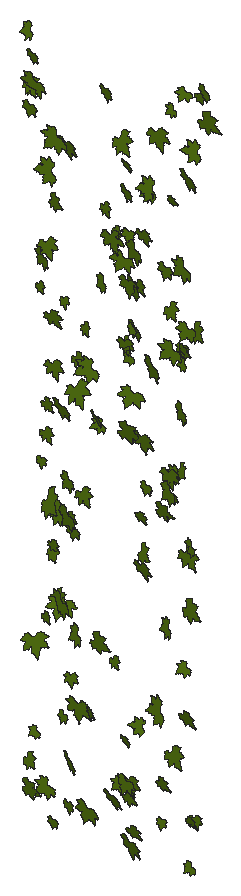
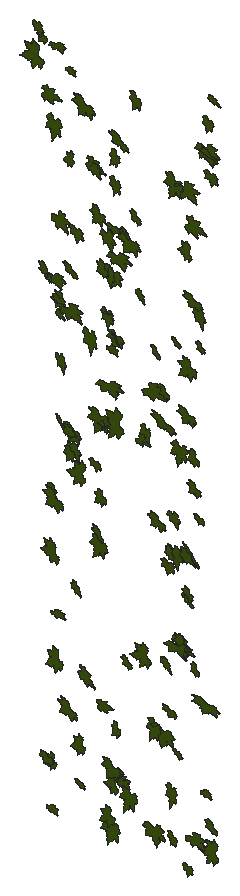
# SketchUp Ruby script. Lengths in inches.
U = 1.inch
M = Sketchup.active_model
def pt(a) = Geom::Point3d.new(a.map { |v| v * U })
def face(e, loops, mat)
  f = e.add_face(loops[0].map { |a| pt(a) })
  loops[1..].each { |l| e.add_face(l.map { |a| pt(a) }).erase! }
  f.material = f.back_material = mat if mat
  f
end
# faces: each face lists its corners as indices into pts; further lists are holes
def faces(e, pts, list, mat = nil) = list.each { |f| face(e, (f[0].is_a?(Array) ? f : [f]).map { |l| l.map { |i| pts[i] } }, mat) }
# xy, xz, yz: faces in a plane at the given z, y or x. An outline is a flat list of corners, or four numbers for a rectangle; further outlines are holes
def ring(l) = l.size == 4 ? [[l[0], l[1]], [l[2], l[1]], [l[2], l[3]], [l[0], l[3]]] : l.each_slice(2).to_a
def flat(e, list, mat, &to3) = list.each { |f| face(e, (f[0].is_a?(Array) ? f : [f]).map { |l| ring(l).map { |u, v| to3.(u, v) } }, mat) }
def xy(e, z, list, mat = nil) = flat(e, list, mat) { |x, y| [x, y, z] }
def xz(e, y, list, mat = nil) = flat(e, list, mat) { |x, z| [x, y, z] }
def yz(e, x, list, mat = nil) = flat(e, list, mat) { |y, z| [x, y, z] }
def lines(e, pts, list) = list.each { |a, b| e.add_line(pt(pts[a]), pt(pts[b])) }
# prism: a flat outline (further loops are holes) pulled along v
def prism(e, loops, v, mat = nil)
  f = face(e, loops, mat); d = Geom::Vector3d.new(v.map { |x| x * U })
  f.pushpull(f.normal.samedirection?(d) ? d.length : -d.length)
end
def box(e, o, s, mat = nil) = prism(e, [[o, [o[0] + s[0], o[1], o[2]], [o[0] + s[0], o[1] + s[1], o[2]], [o[0], o[1] + s[1], o[2]]]], [0, 0, s[2]], mat)
def at(x, y, z, deg = 0) = Geom::Transformation.translation(pt([x, y, z])) * Geom::Transformation.rotation(ORIGIN, Z_AXIS, deg.degrees)
def axes(o, x, y, z) = Geom::Transformation.new([*x, 0, *y, 0, *z, 0, *pt(o).to_a, 1])
def part(name) = M.definitions.add(name)
# library, detail: a bought-in or finely detailed component or shape, given as its bounding box
def library(name, o, s) = part(name).tap { |d| box(d.entities, o, s) }
def detail(e, o, s) = box(e.add_group.entities, o, s)
def put(e, d, t, mat = nil) = e.add_instance(d, t).tap { |i| i.material = mat if mat }
def group(e, t, mat = nil) = e.add_group.tap { |g| g.transformation = t; g.material = mat if mat }.entities
root = M.entities
M.materials.add("[Vegetation Blur 03]").color = [83, 114, 18]
c1 = part("ivy")
xy(c1.entities,0,[[0.782,0,0.786,0,0.787,0.005,0.789,0.009,0.821,0.072,0.875,0.147,1.001,0.272,1.073,0.331,1.137,0.363,1.178,0.379,1.223,0.384,1.272,0.383,1.311,0.374,1.36,0.355,1.399,0.334,1.491,0.285,1.541,0.244,1.583,0.199,1.617,0.15,1.64,0.128,1.662,0.115,1.717,0.105,1.745,0.093,1.784,0.054,1.819,0.057,1.854,0.064,1.882,0.075,1.896,0.074,1.91,0.071,1.937,0.063,1.964,0.053,1.99,0.038,2.016,0.015,2.034,0.002,2.04,0,2.038,0.003,2.036,0.007,2.033,0.038,2.036,0.068,2.045,0.1,2.055,0.116,2.064,0.123,2.077,0.129,2.088,0.129,2.106,0.132,2.118,0.13,2.179,0.132,2.207,0.133,2.225,0.133,2.242,0.138,2.22,0.162,2.207,0.186,2.206,0.213,2.212,0.236,2.228,0.262,2.247,0.274,2.298,0.283,2.355,0.294,2.37,0.296,2.376,0.295,2.377,0.3,2.377,0.303,2.385,0.329,2.411,0.37,2.426,0.392,2.449,0.407,2.511,0.426,2.561,0.444,2.619,0.466,2.589,0.469,2.561,0.476,2.501,0.5,2.449,0.516,2.424,0.523,2.401,0.535,2.377,0.556,2.372,0.568,2.36,0.575,2.268,0.586,2.225,0.592,2.207,0.599,2.194,0.61,2.143,0.65,2.13,0.664,2.122,0.682,2.123,0.7,2.13,0.719,2.148,0.75,2.17,0.781,2.195,0.807,2.221,0.828,2.284,0.874,2.291,0.88,2.288,0.887,2.276,0.9,2.267,0.916,2.265,0.933,2.273,0.967,2.292,1.002,2.313,1.03,2.334,1.054,2.348,1.067,2.358,1.074,2.363,1.076,2.362,1.081,2.35,1.094,2.347,1.11,2.35,1.143,2.359,1.18,2.385,1.254,2.415,1.324,2.448,1.393,2.45,1.4,2.446,1.398,2.44,1.394,2.427,1.383,2.402,1.36,2.376,1.339,2.345,1.324,2.305,1.309,2.282,1.303,2.273,1.306,2.245,1.294,2.212,1.287,2.187,1.291,2.163,1.301,2.142,1.316,2.134,1.327,2.124,1.325,2.09,1.292,2.053,1.259,2.014,1.234,1.973,1.215,1.954,1.21,1.931,1.208,1.909,1.212,1.893,1.22,1.879,1.233,1.872,1.248,1.867,1.281,1.864,1.319,1.821,1.258,1.773,1.197,1.726,1.141,1.698,1.121,1.679,1.116,1.666,1.117,1.647,1.122,1.632,1.129,1.62,1.141,1.617,1.154,1.617,1.219,1.621,1.254,1.623,1.268,1.623,1.281,1.618,1.314,1.606,1.346,1.603,1.375,1.607,1.403,1.603,1.467,1.599,1.499,1.605,1.525,1.614,1.552,1.629,1.577,1.635,1.589,1.629,1.587,1.618,1.582,1.596,1.566,1.581,1.556,1.568,1.552,1.557,1.55,1.545,1.553,1.531,1.562,1.522,1.572,1.504,1.591,1.486,1.611,1.474,1.631,1.457,1.666,1.455,1.684,1.457,1.698,1.452,1.715,1.444,1.728,1.424,1.754,1.419,1.772,1.423,1.786,1.434,1.819,1.444,1.848,1.446,1.855,1.44,1.861,1.43,1.867,1.386,1.904,1.349,1.948,1.326,1.973,1.31,1.995,1.288,2.048,1.284,2.153,1.287,2.254,1.284,2.255,1.282,2.253,1.278,2.247,1.274,2.237,1.266,2.216,1.226,2.125,1.208,2.076,1.184,2.033,1.155,1.984,1.135,1.942,1.111,1.899,1.083,1.861,1.053,1.85,1.059,1.83,1.061,1.809,1.056,1.79,1.049,1.767,1.04,1.749,1.018,1.733,0.994,1.726,0.942,1.734,0.95,1.6875,0.944,1.645,0.932,1.608,0.911,1.585,0.881,1.58,0.854,1.582,0.828,1.588,0.785,1.618,0.773,1.625,0.775,1.614,0.779,1.598,0.796,1.502,0.818,1.402,0.861,1.283,0.882,1.224,0.894,1.174,0.892,1.148,0.886,1.123,0.881,1.107,0.872,1.099,0.849,1.094,0.818,1.092,0.789,1.098,0.762,1.107,0.753,1.113,0.721,1.139,0.698,1.163,0.678,1.194,0.665,1.224,0.628,1.28,0.612,1.312,0.606,1.327,0.606,1.314,0.599,1.282,0.594,1.267,0.581,1.256,0.544,1.245,0.512,1.244,0.473,1.249,0.444,1.256,0.382,1.288,0.339,1.306,0.324,1.316,0.317,1.324,0.309,1.326,0.27,1.314,0.227,1.313,0.185,1.3125,0.152,1.317,0.122,1.328,0.092,1.345,0.073,1.353,0.079,1.338,0.092,1.308,0.117,1.249,0.13,1.215,0.139,1.164,0.147,1.148,0.157,1.136,0.163,1.122,0.174,1.086,0.177,1.067,0.182,1.054,0.186,1.043,0.191,1.038,0.211,1.028,0.237,1.005,0.25,0.974,0.253,0.96,0.25,0.944,0.242,0.914,0.243,0.906,0.249,0.902,0.26,0.894,0.289,0.88,0.307,0.873,0.322,0.862,0.364,0.799,0.403,0.738,0.431,0.709,0.439,0.691,0.441,0.678,0.4375,0.66,0.428,0.645,0.394,0.623,0.303,0.594,0.255,0.581,0.214,0.577,0.179,0.573,0.173,0.568,0.175,0.561,0.167,0.55,0.141,0.523,0.113,0.503,0.077,0.49,0.045,0.486,0.026,0.485,0.019,0.486,0.011,0.483,0,0.471,0.014,0.467,0.044,0.455,0.058,0.447,0.07,0.438,0.097,0.411,0.125,0.394,0.158,0.377,0.174,0.366,0.182,0.359,0.185,0.361,0.242,0.331,0.253,0.316,0.258,0.303,0.262,0.283,0.274,0.278,0.308,0.274,0.341,0.252,0.366,0.226,0.366,0.222,0.37,0.22,0.38,0.221,0.395,0.221,0.425,0.216,0.45,0.207,0.465,0.192,0.473,0.178,0.484,0.15,0.489,0.116,0.483,0.089,0.468,0.058,0.45,0.035,0.435,0.018,0.429,0.011,0.434,0.012,0.438,0.014,0.469,0.019,0.542,0.016,0.581,0.015,0.612,0.027,0.68,0.055,0.696,0.057,0.712,0.052,0.73,0.045,0.741,0.036,0.766,0.014]])
put(root,c1,axes([22.26,173.7,49.1875],[0.2034,-0.19719,-0.25526],[-0.32297,-0.00076,-0.17132],[-0.05192,-0.76775,0.06573]),"[Vegetation Blur 03]")
put(root,c1,axes([21.79,173.7,44.77],[0.4277,-0.13208,-0.01923],[-0.02433,-0.00684,-0.35292],[-0.0639,-0.88143,0.00562]),"[Vegetation Blur 03]")
put(root,c1,axes([21.72,173.7,8.45],[0.18478,0.02807,0.2907],[0.35178,-0.14758,-0.1467],[-0.05752,-0.81244,0.03669]),"[Vegetation Blur 03]")
put(root,c1,axes([21.94,173.7,46.46],[0.60025,-0.11632,-0.20653],[-0.25299,0.02521,-0.49198],[-0.05685,-1.34025,0.00867]),"[Vegetation Blur 03]")
put(root,c1,axes([21.68,173.7,45.55],[0.34233,0.0367,0.25351],[0.30852,-0.16299,-0.27378],[-0.04025,-0.93715,0.05755]),"[Vegetation Blur 03]")
put(root,c1,axes([21.74,173.7,6.73],[0.10484,-0.11239,0.45286],[0.55605,-0.06423,-0.08825],[-0.04094,-1.16025,-0.03898]),"[Vegetation Blur 03]")
put(root,c1,axes([22,173.7,47.62],[0.38177,-0.16884,0.00908],[0.01686,0.05275,-0.31784],[-0.08106,-0.78418,-0.02334]),"[Vegetation Blur 03]")
put(root,c1,axes([22.47,173.7,10.74],[0.21979,-0.07452,-0.15702],[-0.1954,-0.04663,-0.1787],[-0.01213,-0.59927,0.03343]),"[Vegetation Blur 03]")
put(root,c1,axes([21.59,173.7,15.34],[0.58242,0.07305,0.2372],[0.29248,-0.20649,-0.46835],[-0.01349,-1.32342,0.08617]),"[Vegetation Blur 03]")
put(root,c1,axes([22.71,173.7,37.14],[0.45147,-0.25025,-0.22719],[-0.26949,0.14362,-0.38159],[-0.1402,-1.08195,0.00189]),"[Vegetation Blur 03]")
put(root,c1,axes([22.51,173.7,34.78],[0.19571,-0.04059,0.18321],[0.21938,-0.10557,-0.15978],[-0.05153,-0.6037,0.01562]),"[Vegetation Blur 03]")
put(root,c1,axes([22.6,173.7,25.49],[0.2893,-0.06946,0.05279],[0.06075,-0.07196,-0.23668],[-0.04039,-0.60575,0.02206]),"[Vegetation Blur 03]")
put(root,c1,axes([23.02,173.7,8.21],[0.3982,-0.07833,-0.27853],[-0.34327,-0.06231,-0.32413],[-0.0091,-1.07738,0.039]),"[Vegetation Blur 03]")
put(root,c1,axes([23.625,173.7,42.125],[0.18243,-0.13935,-0.48722],[-0.59996,0.02639,-0.15082],[-0.03212,-1.28429,0.04976]),"[Vegetation Blur 03]")
put(root,c1,axes([22.87,173.7,16.84],[0.19414,-0.08015,0.20136],[0.24242,-0.09451,-0.1616],[-0.0602,-0.6391,-0.00136]),"[Vegetation Blur 03]")
put(root,c1,axes([22.71,173.7,26.84],[0.30004,-0.03578,0.23182],[0.28092,-0.09842,-0.24458],[-0.04545,-0.84451,0.01868]),"[Vegetation Blur 03]")
put(root,c1,axes([22.82,173.7,28.4375],[0.23733,-0.08095,0.26556],[0.32364,-0.07275,-0.19614],[-0.05179,-0.82556,-0.00876]),"[Vegetation Blur 03]")
put(root,c1,axes([22.6,173.7,37.21],[0.44354,0.00148,0.25414],[0.30752,-0.17731,-0.35733],[-0.04893,-1.101,0.05789]),"[Vegetation Blur 03]")
put(root,c1,axes([23.4375,173.7,43.99],[0.532,-0.08529,-0.32199],[-0.3962,-0.04622,-0.4341],[-0.01987,-1.36215,0.03489]),"[Vegetation Blur 03]")
put(root,c1,axes([22.79,173.7,22.68],[0.16553,0.17765,0.51158],[0.60894,-0.40708,-0.109],[-0.17196,-1.2705,0.10646]),"[Vegetation Blur 03]")
put(root,c1,axes([23.31,173.7,6.07],[0.31854,-0.11206,-0.01065],[-0.01233,0.01101,-0.26373],[-0.05462,-0.65595,-0.00261]),"[Vegetation Blur 03]")
put(root,c1,axes([23.23,173.7,20.93],[0.24085,-0.07286,0.19486],[0.23769,-0.04913,-0.19858],[-0.04198,-0.69616,-0.00638]),"[Vegetation Blur 03]")
put(root,c1,axes([23.95,173.7,23.6875],[0.31165,-0.23246,-0.38206],[-0.4746,0.04633,-0.26229],[-0.08166,-1.15634,0.0663]),"[Vegetation Blur 03]")
put(root,c1,axes([22.91,173.7,33.35],[0.40049,-0.10291,0.28569],[0.35224,0.02026,-0.32774],[-0.03114,-1.09438,-0.03293]),"[Vegetation Blur 03]")
put(root,c1,axes([23.2,173.7,20.47],[0.2517,0.01272,0.24338],[0.28699,-0.2291,-0.19581],[-0.08127,-0.76965,0.06231]),"[Vegetation Blur 03]")
put(root,c1,axes([23,173.7,30.8],[0.46612,-0.06322,0.21313],[0.25778,-0.10592,-0.38046],[-0.05188,-1.09436,0.02451]),"[Vegetation Blur 03]")
put(root,c1,axes([23.35,173.7,39.48],[0.11949,-0.05949,0.35767],[0.43416,-0.12523,-0.09989],[-0.06637,-0.92633,-0.00946]),"[Vegetation Blur 03]")
put(root,c1,axes([23.76,173.7,18.71],[0.56265,-0.26157,-0.25412],[-0.30853,0.09554,-0.47049],[-0.13384,-1.31983,0.01631]),"[Vegetation Blur 03]")
put(root,c1,axes([23.4375,173.7,18.27],[0.61939,0.05734,-0.0417],[-0.04546,-0.22498,-0.49845],[0.03634,-1.25897,0.08717]),"[Vegetation Blur 03]")
put(root,c1,axes([23.58,173.7,17.87],[0.12985,0.03067,0.35023],[0.42444,-0.14892,-0.10276],[-0.06505,-0.91052,0.02861]),"[Vegetation Blur 03]")
put(root,c1,axes([23.57,173.7,29.13],[0.58072,-0.2362,-0.06513],[-0.0644,0.17074,-0.47989],[-0.12408,-1.1941,-0.05574]),"[Vegetation Blur 03]")
put(root,c1,axes([24.06,173.7,12.16],[0.30014,-0.14068,-0.03498],[-0.05049,-0.06238,-0.24906],[-0.06295,-0.62077,0.03295]),"[Vegetation Blur 03]")
put(root,c1,axes([24,173.7,34.61],[0.25172,-0.04798,0.1294],[0.15152,-0.12662,-0.20371],[-0.0522,-0.59895,0.0327]),"[Vegetation Blur 03]")
put(root,c1,axes([24.1,173.7,23.53],[0.559,-0.25408,-0.226],[-0.26774,0.14716,-0.46713],[-0.14227,-1.27524,-0.00888]),"[Vegetation Blur 03]")
put(root,c1,axes([24.28,173.7,25.35],[0.41365,-0.19736,-0.16762],[-0.20533,0.04633,-0.34609],[-0.09602,-0.94924,0.01796]),"[Vegetation Blur 03]")
put(root,c1,axes([23.8,173.7,43.49],[0.6079,-0.24736,0.08777],[0.11732,0.08596,-0.50313],[-0.11068,-1.26744,-0.05125]),"[Vegetation Blur 03]")
put(root,c1,axes([24.22,173.7,7.27],[0.34382,-0.15266,0.07768],[0.0934,-0.03785,-0.28706],[-0.07642,-0.73315,-0.00136]),"[Vegetation Blur 03]")
put(root,c1,axes([24.26,173.7,10.05],[0.51362,-0.33546,-0.11294],[-0.11227,0.20752,-0.43703],[-0.18199,-1.07476,-0.04914]),"[Vegetation Blur 03]")
put(root,c1,axes([24.29,173.7,14.22],[0.36114,-0.04689,0.10699],[0.12628,-0.12494,-0.29255],[-0.0419,-0.78067,0.04039]),"[Vegetation Blur 03]")
put(root,c1,axes([24.45,173.7,22.66],[0.10493,-0.03643,0.24088],[0.29195,-0.08918,-0.08683],[-0.04677,-0.63839,-0.00162]),"[Vegetation Blur 03]")
put(root,c1,axes([24.41,173.7,22.42],[0.40755,-0.11351,-0.00014],[0.00098,0.01751,-0.33557],[-0.05515,-0.83847,-0.00699]),"[Vegetation Blur 03]")
put(root,c1,axes([25.03,173.7,17.2],[0.33509,-0.2609,-0.26753],[-0.3303,0.08476,-0.28857],[-0.12012,-0.96089,0.04719]),"[Vegetation Blur 03]")
put(root,c1,axes([24.67,173.7,31.48],[0.21376,-0.00368,0.2636],[0.3197,-0.11113,-0.17293],[-0.04601,-0.78924,0.02312]),"[Vegetation Blur 03]")
put(root,c1,axes([24.4,173.7,13.03],[0.66487,-0.12258,0.05657],[0.06821,-0.03171,-0.54475],[-0.06083,-1.37523,0.00752]),"[Vegetation Blur 03]")
put(root,c1,axes([24.24,173.7,29.74],[0.49312,0.07516,0.37451],[0.45503,-0.28887,-0.38996],[-0.06962,-1.3557,0.10386]),"[Vegetation Blur 03]")
put(root,c1,axes([24.85,173.7,24.2],[0.35229,-0.00554,0.29733],[0.36145,-0.12544,-0.28562],[-0.04568,-1.0353,0.03302]),"[Vegetation Blur 03]")
put(root,c1,axes([25.79,173.7,32.11],[0.3559,-0.06669,-0.38571],[-0.47242,-0.14005,-0.28653],[0.03508,-1.20938,0.05445]),"[Vegetation Blur 03]")
put(root,c1,axes([25.12,173.7,7.72],[0.62299,-0.15418,-0.12642],[-0.15294,0.05244,-0.51207],[-0.07884,-1.31998,-0.00558]),"[Vegetation Blur 03]")
put(root,c1,axes([25.27,173.7,33.45],[0.20111,-0.0492,0.23305],[0.27447,-0.17313,-0.16352],[-0.08231,-0.69755,0.02415]),"[Vegetation Blur 03]")
put(root,c1,axes([25.21,173.7,13.0625],[0.49941,-0.26714,0.04177],[0.06827,0.12648,-0.4165],[-0.1217,-1.02529,-0.06226]),"[Vegetation Blur 03]")
put(root,c1,axes([26.49,173.7,28.98],[0.19807,-0.04882,-0.25327],[-0.31096,-0.06252,-0.16009],[0.01294,-0.755,0.02963]),"[Vegetation Blur 03]")
put(root,c1,axes([25.86,173.7,29.22],[0.42582,-0.25778,-0.01572],[0.00049,0.14225,-0.35818],[-0.12674,-0.86554,-0.05419]),"[Vegetation Blur 03]")
put(root,c1,axes([26.57,173.7,36.92],[0.29115,-0.21346,-0.2217],[-0.27097,0.0878,-0.25032],[-0.10549,-0.81469,0.03111]),"[Vegetation Blur 03]")
put(root,c1,axes([25.82,173.7,16.21],[0.18573,-0.07263,0.44986],[0.55141,-0.04477,-0.15278],[-0.03192,-1.19609,-0.0216]),"[Vegetation Blur 03]")
put(root,c1,axes([26.42,173.7,47.22],[0.42985,-0.21428,0.06487],[0.08397,0.02008,-0.36019],[-0.10055,-0.89931,-0.0235]),"[Vegetation Blur 03]")
put(root,c1,axes([26.43,173.7,40.5],[0.26598,-0.07146,0.22657],[0.27016,-0.13937,-0.21816],[-0.07275,-0.7788,0.01825]),"[Vegetation Blur 03]")
put(root,c1,axes([26.61,173.7,8.75],[0.57489,-0.26657,0.03866],[0.06843,0.18847,-0.47339],[-0.11976,-1.17196,-0.08492]),"[Vegetation Blur 03]")
put(root,c1,axes([26.42,173.7,39.15],[0.58643,-0.10608,0.2337],[0.28408,-0.0778,-0.48036],[-0.06289,-1.34069,0.00938]),"[Vegetation Blur 03]")
put(root,c1,axes([26.98,173.7,15.82],[0.22624,-0.03067,0.2044],[0.24637,-0.10398,-0.18409],[-0.04741,-0.6867,0.01875]),"[Vegetation Blur 03]")
put(root,c1,axes([27.58,173.7,9.77],[0.29889,-0.0519,-0.2268],[-0.27904,-0.05258,-0.24304],[-0.001,-0.83818,0.02929]),"[Vegetation Blur 03]")
put(root,c1,axes([27.17,173.7,39.43],[0.18943,-0.02258,0.18927],[0.22327,-0.15119,-0.15168],[-0.06367,-0.59736,0.03124]),"[Vegetation Blur 03]")
put(root,c1,axes([27.38,173.7,38.5625],[0.53942,-0.03341,-0.15907],[-0.19556,-0.07489,-0.43924],[-0.00287,-1.17788,0.03244]),"[Vegetation Blur 03]")
put(root,c1,axes([27.11,173.7,44.22],[0.34036,0.06769,0.40355],[0.48921,-0.24292,-0.26842],[-0.07909,-1.21115,0.07639]),"[Vegetation Blur 03]")
put(root,c1,axes([27.62,173.7,9.97],[0.51001,-0.14732,-0.08686],[-0.10909,-0.02593,-0.41973],[-0.06746,-1.07179,0.02209]),"[Vegetation Blur 03]")
put(root,c1,axes([27.78,173.7,33.21],[0.05918,0.07636,0.27369],[0.32495,-0.20144,-0.03796],[-0.0908,-0.67116,0.04253]),"[Vegetation Blur 03]")
put(root,c1,axes([27.48,173.7,33.69],[0.45211,-0.0957,0.11404],[0.13937,-0.02195,-0.37092],[-0.04759,-0.97354,-0.00285]),"[Vegetation Blur 03]")
put(root,c1,axes([27.7,173.7,11.97],[0.28812,-0.17967,0.12477],[0.15963,0.01216,-0.24278],[-0.07425,-0.67108,-0.0378]),"[Vegetation Blur 03]")
put(root,c1,axes([27.71,173.7,42.25],[0.44121,-0.22953,-0.01023],[-0.00431,0.06987,-0.3705],[-0.11216,-0.9056,-0.026]),"[Vegetation Blur 03]")
put(root,c1,axes([27.84,173.7,39.79],[0.32765,-0.02489,0.01881],[0.02157,-0.07508,-0.26601],[-0.01455,-0.67173,0.02903]),"[Vegetation Blur 03]")
put(root,c1,axes([28.2,173.7,33.24],[0.24945,-0.08617,-0.15972],[-0.19859,-0.02674,-0.20432],[-0.02483,-0.6519,0.02949]),"[Vegetation Blur 03]")
put(root,c1,axes([27.73,173.7,43.5625],[0.34754,-0.2147,0.09746],[0.13272,0.06991,-0.29103],[-0.08677,-0.75297,-0.05481]),"[Vegetation Blur 03]")
put(root,c1,axes([27.86,173.7,31.3],[0.55742,0.02012,-0.13001],[-0.15728,-0.13301,-0.4524],[0.0271,-1.18554,0.04855]),"[Vegetation Blur 03]")
put(root,c1,axes([27.61,173.7,37.24],[0.58629,-0.17522,0.04019],[0.04988,0.00183,-0.48347],[-0.08478,-1.21072,-0.00655]),"[Vegetation Blur 03]")
put(root,c1,axes([27.53,173.7,28.28],[0.20202,-0.16973,0.51163],[0.63222,0.07532,-0.16235],[0.00985,-1.35325,-0.07321]),"[Vegetation Blur 03]")
put(root,c1,axes([27.85,173.7,8.5],[0.13655,-0.05783,0.35944],[0.43753,-0.10617,-0.1134],[-0.05764,-0.9429,-0.00928]),"[Vegetation Blur 03]")
put(root,c1,axes([27.625,173.7,9.74],[0.52125,-0.12471,0.19571],[0.23821,-0.0569,-0.42827],[-0.06661,-1.17932,-0.00003]),"[Vegetation Blur 03]")
put(root,c1,axes([28.33,173.7,34.86],[0.28246,-0.12607,-0.06429],[-0.08477,-0.04633,-0.23378],[-0.05266,-0.60166,0.03147]),"[Vegetation Blur 03]")
put(root,c1,axes([27.72,173.7,6.72],[0.66178,-0.29714,0.00728],[0.02239,0.12543,-0.55031],[-0.14293,-1.35615,-0.0525]),"[Vegetation Blur 03]")
put(root,c1,axes([28.29,173.7,39.5],[0.50423,-0.25138,-0.23976],[-0.28758,0.12452,-0.42338],[-0.1361,-1.1944,0.00632]),"[Vegetation Blur 03]")
put(root,c1,axes([28.2,173.7,37.44],[0.499,-0.30069,-0.16614],[-0.19194,0.14146,-0.42426],[-0.16109,-1.09995,-0.00914]),"[Vegetation Blur 03]")
put(root,c1,axes([28.24,173.7,35.02],[0.4623,-0.23108,-0.11744],[-0.13279,0.12742,-0.38762],[-0.12523,-0.98816,-0.02252]),"[Vegetation Blur 03]")
put(root,c1,axes([28,173.7,6.9],[0.29257,-0.13243,0.26003],[0.3239,0.04481,-0.23915],[-0.02726,-0.88901,-0.05079]),"[Vegetation Blur 03]")
put(root,c1,axes([29.22,173.7,13.41],[0.05855,-0.11186,-0.32035],[-0.39567,-0.06136,-0.0448],[0.02177,-0.81436,0.04738]),"[Vegetation Blur 03]")
put(root,c1,axes([28.45,173.7,36.92],[0.26922,-0.1042,0.25304],[0.30661,-0.09593,-0.2235],[-0.06845,-0.83952,-0.00587]),"[Vegetation Blur 03]")
put(root,c1,axes([28.54,173.7,24.4],[0.28875,-0.1223,0.18363],[0.229,0.01809,-0.23796],[-0.04139,-0.75306,-0.03554]),"[Vegetation Blur 03]")
put(root,c1,axes([28.32,173.7,28.96],[0.63148,-0.16792,0.0994],[0.12538,0.04433,-0.51879],[-0.07597,-1.32267,-0.03001]),"[Vegetation Blur 03]")
put(root,c1,axes([28.4375,173.7,21.86],[0.52924,-0.21641,0.13482],[0.17446,0.07604,-0.43695],[-0.08896,-1.13835,-0.05482]),"[Vegetation Blur 03]")
put(root,c1,axes([28.75,173.7,22.02],[0.07963,0.08394,0.36792],[0.43963,-0.2386,-0.05481],[-0.10777,-0.91131,0.04824]),"[Vegetation Blur 03]")
put(root,c1,axes([29.3,173.7,42.93],[0.3287,-0.1611,-0.24597],[-0.30329,0.03864,-0.27395],[-0.07054,-0.91688,0.03167]),"[Vegetation Blur 03]")
put(root,c1,axes([28.59,173.7,39.98],[0.42324,-0.15513,0.17492],[0.21736,0.00516,-0.3496],[-0.06611,-0.97622,-0.02964]),"[Vegetation Blur 03]")
put(root,c1,axes([29.75,173.7,43.27],[0.20332,-0.17652,-0.4378],[-0.54125,0.03497,-0.16965],[-0.04646,-1.17997,0.06046]),"[Vegetation Blur 03]")
put(root,c1,axes([29.02,173.7,26.42],[0.35274,-0.11868,-0.02991],[-0.03922,-0.02703,-0.29129],[-0.05595,-0.72928,0.01566]),"[Vegetation Blur 03]")
put(root,c1,axes([29.26,173.7,33.5],[0.58606,-0.32249,-0.17371],[-0.19607,0.18401,-0.49434],[-0.17725,-1.2698,-0.02752]),"[Vegetation Blur 03]")
put(root,c1,axes([30.19,173.7,15.02],[0.29249,-0.26424,-0.46367],[-0.56799,0.1604,-0.25303],[-0.12902,-1.30512,0.06278]),"[Vegetation Blur 03]")
put(root,c1,axes([29.22,173.7,45.69],[0.56787,-0.08069,0.24242],[0.2938,-0.10677,-0.464],[-0.05873,-1.31444,0.02281]),"[Vegetation Blur 03]")
put(root,c1,axes([29.98,173.7,8.3],[0.28663,-0.07213,0.05383],[0.05877,-0.11436,-0.23255],[-0.04609,-0.59433,0.03821]),"[Vegetation Blur 03]")
put(root,c1,axes([30.63,173.7,19.48],[0.25494,-0.21897,-0.29058],[-0.35433,0.12452,-0.22182],[-0.11199,-0.89248,0.04035]),"[Vegetation Blur 03]")
put(root,c1,axes([29.875,173.7,10.08],[0.21568,-0.13397,0.30172],[0.37321,-0.01782,-0.17894],[-0.04036,-0.88058,-0.04228]),"[Vegetation Blur 03]")
put(root,c1,axes([30.06,173.7,38.82],[0.45457,-0.14322,-0.01986],[-0.02603,-0.01905,-0.37516],[-0.06898,-0.93657,0.01067]),"[Vegetation Blur 03]")
put(root,c1,axes([29.93,173.7,24.8],[0.10325,-0.14377,0.42811],[0.52829,-0.03594,-0.08677],[-0.03077,-1.09956,-0.05314]),"[Vegetation Blur 03]")
put(root,c1,axes([30.59,173.7,34.76],[0.44525,-0.05596,-0.30949],[-0.38019,-0.06333,-0.36251],[-0.0007,-1.20185,0.03351]),"[Vegetation Blur 03]")
put(root,c1,axes([30.5,173.7,27.08],[0.46711,-0.27655,-0.25561],[-0.31156,0.09667,-0.39569],[-0.13813,-1.15324,0.02812]),"[Vegetation Blur 03]")
put(root,c1,axes([30.82,173.7,47.71],[0.23115,-0.1069,-0.165],[-0.20647,-0.0259,-0.19002],[-0.03067,-0.63139,0.03573]),"[Vegetation Blur 03]")
put(root,c1,axes([31.19,173.7,27.94],[0.13432,-0.12713,-0.31462],[-0.38869,0.03529,-0.11278],[-0.03669,-0.83931,0.04291]),"[Vegetation Blur 03]")
put(root,c1,axes([30.1,173.7,27.48],[0.52424,-0.12738,0.15619],[0.18843,-0.07357,-0.4307],[-0.07036,-1.14606,0.01029]),"[Vegetation Blur 03]")
put(root,c1,axes([30.5,173.7,26.375],[0.34163,-0.14558,0.05444],[0.07406,0.06471,-0.28235],[-0.063,-0.71335,-0.03672]),"[Vegetation Blur 03]")
put(root,c1,axes([30.31,173.7,36.14],[0.2559,0.03571,0.2999],[0.36108,-0.20047,-0.20147],[-0.07032,-0.89939,0.05682]),"[Vegetation Blur 03]")
put(root,c1,axes([30.62,173.7,42.23],[0.11718,-0.12684,0.22641],[0.28293,-0.00575,-0.09804],[-0.02661,-0.61967,-0.04543]),"[Vegetation Blur 03]")
put(root,c1,axes([30.28,173.7,11.83],[0.38921,-0.01895,0.37093],[0.44943,-0.16908,-0.31546],[-0.06835,-1.21968,0.03797]),"[Vegetation Blur 03]")
put(root,c1,axes([31.32,173.7,39.57],[0.45075,-0.16208,-0.3284],[-0.40131,0.07789,-0.37294],[-0.08406,-1.24093,0.01948]),"[Vegetation Blur 03]")
put(root,c1,axes([31.59,173.7,34.06],[0.16581,-0.12598,-0.20066],[-0.24842,0.03821,-0.1405],[-0.04988,-0.60905,0.03269]),"[Vegetation Blur 03]")
put(root,c1,axes([31.28,173.7,31.63],[0.43303,-0.27941,-0.22313],[-0.26455,0.14367,-0.37028],[-0.1523,-1.044,0.00876]),"[Vegetation Blur 03]")
put(root,c1,axes([31.14,173.7,34.65],[0.34203,-0.05341,0.04309],[0.05121,-0.04542,-0.27956],[-0.02898,-0.71072,0.01463]),"[Vegetation Blur 03]")
put(root,c1,axes([31.36,173.7,48.8125],[0.33694,0.0048,-0.1079],[-0.13035,-0.11296,-0.27192],[0.0222,-0.7362,0.04102]),"[Vegetation Blur 03]")
put(root,c1,axes([31.16,173.7,27.48],[0.09035,0.0602,0.28294],[0.33236,-0.23291,-0.06289],[-0.10289,-0.69949,0.04529]),"[Vegetation Blur 03]")
put(root,c1,axes([31.61,173.7,17.49],[0.26178,-0.07777,-0.19292],[-0.23918,-0.11506,-0.20887],[0.01,-0.71663,0.05447]),"[Vegetation Blur 03]")
put(root,c1,axes([31.41,173.7,36.04],[0.46854,-0.05722,-0.15501],[-0.19159,-0.07548,-0.38134],[-0.0119,-1.03762,0.03629]),"[Vegetation Blur 03]")
put(root,c1,axes([31.31,173.7,34.125],[0.08947,-0.09548,0.30203],[0.3696,-0.08246,-0.07703],[-0.05008,-0.77914,-0.02886]),"[Vegetation Blur 03]")
put(root,c1,axes([31.32,173.7,44.42],[0.59182,-0.28218,-0.07799],[-0.07654,0.18572,-0.49252],[-0.14859,-1.21956,-0.05695]),"[Vegetation Blur 03]")
put(root,c1,axes([31.89,173.7,6.625],[0.26116,-0.07939,-0.16142],[-0.20062,-0.0401,-0.21311],[-0.01886,-0.67295,0.03174]),"[Vegetation Blur 03]")
put(root,c1,axes([31.9,173.7,24.29],[0.32555,-0.21056,-0.17248],[-0.21105,0.06347,-0.27751],[-0.10292,-0.79617,0.02349]),"[Vegetation Blur 03]")
put(root,c1,axes([31.21,173.7,14.29],[0.35259,-0.1904,0.31199],[0.38853,0.00444,-0.29204],[-0.06112,-1.07015,-0.05672]),"[Vegetation Blur 03]")
put(root,c1,axes([32.54,173.7,46.18],[0.12519,-0.10736,-0.42184],[-0.51949,-0.03465,-0.1013],[0.00417,-1.09384,0.04461]),"[Vegetation Blur 03]")
put(root,c1,axes([31.12,173.7,23.15],[0.45704,-0.07073,0.34791],[0.42202,-0.13355,-0.37354],[-0.06933,-1.27915,0.01976]),"[Vegetation Blur 03]")
put(root,c1,axes([31.65,173.7,8.6875],[0.21432,-0.13844,0.2244],[0.28013,0.00181,-0.17803],[-0.04065,-0.71738,-0.04375]),"[Vegetation Blur 03]")
put(root,c1,axes([31.44,173.7,19.93],[0.19345,-0.03327,0.47278],[0.57353,-0.16922,-0.15818],[-0.0831,-1.24533,0.00886]),"[Vegetation Blur 03]")
put(root,c1,axes([31.82,173.7,8.98],[0.33883,-0.03876,0.14234],[0.17237,-0.07132,-0.27636],[-0.03256,-0.78094,0.01817]),"[Vegetation Blur 03]")
put(root,c1,axes([31.92,173.7,35.4],[0.18898,0.02634,0.37085],[0.44381,-0.22984,-0.14807],[-0.09838,-0.98629,0.04441]),"[Vegetation Blur 03]")
put(root,c1,axes([32.21,173.7,48.62],[0.24814,-0.07421,0.13501],[0.16554,-0.02052,-0.20443],[-0.03556,-0.61336,-0.0095]),"[Vegetation Blur 03]")
put(root,c1,axes([32.625,173.7,49.43],[0.36865,-0.17556,-0.1237],[-0.14943,0.05438,-0.30876],[-0.08901,-0.81841,0.00602]),"[Vegetation Blur 03]")
put(root,c1,axes([32.37,173.7,47.01],[0.28018,-0.09633,0.48866],[0.59963,-0.03141,-0.22997],[-0.03369,-1.35996,-0.0293]),"[Vegetation Blur 03]")
